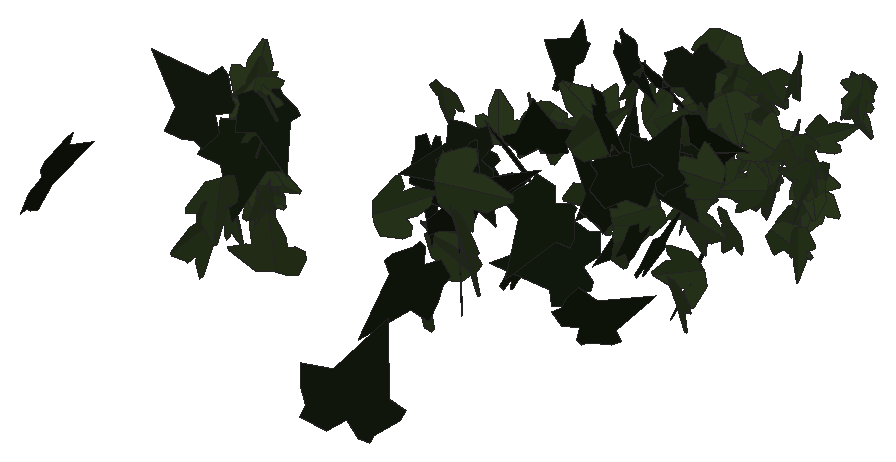
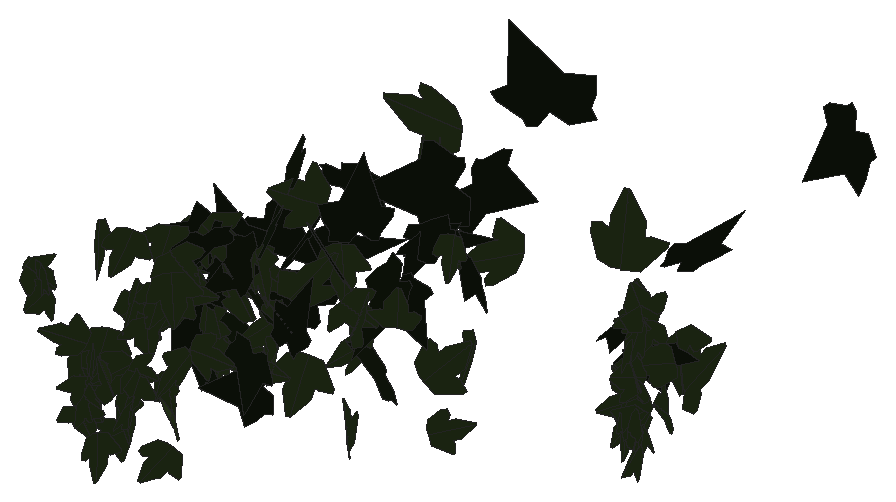
# SketchUp Ruby script. Lengths in inches.
U = 1.inch
M = Sketchup.active_model
def pt(a) = Geom::Point3d.new(a.map { |v| v * U })
def face(e, loops, mat)
  f = e.add_face(loops[0].map { |a| pt(a) })
  loops[1..].each { |l| e.add_face(l.map { |a| pt(a) }).erase! }
  f.material = f.back_material = mat if mat
  f
end
# faces: each face lists its corners as indices into pts; further lists are holes
def faces(e, pts, list, mat = nil) = list.each { |f| face(e, (f[0].is_a?(Array) ? f : [f]).map { |l| l.map { |i| pts[i] } }, mat) }
# xy, xz, yz: faces in a plane at the given z, y or x. An outline is a flat list of corners, or four numbers for a rectangle; further outlines are holes
def ring(l) = l.size == 4 ? [[l[0], l[1]], [l[2], l[1]], [l[2], l[3]], [l[0], l[3]]] : l.each_slice(2).to_a
def flat(e, list, mat, &to3) = list.each { |f| face(e, (f[0].is_a?(Array) ? f : [f]).map { |l| ring(l).map { |u, v| to3.(u, v) } }, mat) }
def xy(e, z, list, mat = nil) = flat(e, list, mat) { |x, y| [x, y, z] }
def xz(e, y, list, mat = nil) = flat(e, list, mat) { |x, z| [x, y, z] }
def yz(e, x, list, mat = nil) = flat(e, list, mat) { |y, z| [x, y, z] }
def lines(e, pts, list) = list.each { |a, b| e.add_line(pt(pts[a]), pt(pts[b])) }
# prism: a flat outline (further loops are holes) pulled along v
def prism(e, loops, v, mat = nil)
  f = face(e, loops, mat); d = Geom::Vector3d.new(v.map { |x| x * U })
  f.pushpull(f.normal.samedirection?(d) ? d.length : -d.length)
end
def box(e, o, s, mat = nil) = prism(e, [[o, [o[0] + s[0], o[1], o[2]], [o[0] + s[0], o[1] + s[1], o[2]], [o[0], o[1] + s[1], o[2]]]], [0, 0, s[2]], mat)
def at(x, y, z, deg = 0) = Geom::Transformation.translation(pt([x, y, z])) * Geom::Transformation.rotation(ORIGIN, Z_AXIS, deg.degrees)
def axes(o, x, y, z) = Geom::Transformation.new([*x, 0, *y, 0, *z, 0, *pt(o).to_a, 1])
def part(name) = M.definitions.add(name)
# library, detail: a bought-in or finely detailed component or shape, given as its bounding box
def library(name, o, s) = part(name).tap { |d| box(d.entities, o, s) }
def detail(e, o, s) = box(e.add_group.entities, o, s)
def put(e, d, t, mat = nil) = e.add_instance(d, t).tap { |i| i.material = mat if mat }
def group(e, t, mat = nil) = e.add_group.tap { |g| g.transformation = t; g.material = mat if mat }.entities
root = M.entities
M.materials.add("efeu1").color = [18, 25, 13]
M.materials.add("efeu2").color = [43, 57, 29]
c1 = part("ivyleaf_10")
p = [[0,0.5,-0.03],[-0.0625,2.02,-0.43],[-0.19,2.01,-0.46],[-0.54,1.05,-0.29],[-0.52,0.625,-0.18],[-0.83,0.76,-0.28],
  [-1.16,0.64,-0.33],[-1.15,0.33,-0.24],[-0.77,-0.39,0.02],[-0.3,-0.51,0.16],[0.04,-0.48,0.23],[-0.02,2.01,-0.4375],
  [-0.06,2.01,-0.43],[0.04,-0.49,0.23],[0.67,-0.49,0.14],[1.38,0.36,-0.2],[1.375,0.51,-0.24],[0.81,0.65,-0.19],
  [0.62,0.59,-0.15],[0.6,1.09,-0.28],[0.5,1.23,-0.31]]
faces(c1.entities,p,[[0,1,2,3,4,5,6,7,8,9,10],[11,12,0,13,14,15,16,17,18,19,20]],"efeu2")
c2 = part("ivyleaf_9")
p = [[1.54,2.16,1.25],[1.36,2.04,1.19],[-0.21,0.99,0.68],[-0.71,1.11,0.82],[-0.85,0.86,0.67],[-0.8,0.17,0.21],
  [-0.9,-0.01,0.1],[-0.67,-0.16,-0.02],[-0.08,-0.08,-0.05],[-0.03,-0.6,-0.4],[0.65,-0.88,-0.66],[0.83,-0.6,-0.49],
  [1.29,-0.42,-0.43],[1.8125,-0.07,-0.26],[1.21,0.44,0.15]]
faces(c2.entities,p,[[0,1,2,3,4,5,6,7,8,9,10,11,12,13,14]],"efeu1")
put(root,c1,axes([585.76,128.17,162.25],[-0.17005,-0.68524,-0.06078],[0.01227,-0.06562,0.70548],[-0.68782,0.16825,0.02761]))
put(root,c1,axes([585.82,127.98,162.4],[0.37144,0.64539,-0.33053],[0.14686,0.29672,0.7444],[0.71007,-0.39897,0.01894]))
put(root,c2,axes([586.1,116.46,164.15],[-0.29886,0.48619,-0.98361],[-0.5513,0.81487,0.57029],[0.94865,0.62673,0.02154]))
put(root,c1,axes([586.01,128.02,157.12],[0.06596,-0.11263,-0.71846],[-0.05388,0.71867,-0.11761],[0.72524,0.06363,0.05661]))
put(root,c1,axes([585.97,128.1875,160],[0.0874,-0.33565,0.67412],[-0.16899,0.65259,0.34684],[-0.73385,-0.19025,0.00041]))
put(root,c2,axes([586.45,125.03,162.97],[-0.48659,-0.88874,-0.04131],[-0.00959,-0.04184,1.01316],[-0.88965,0.48655,0.01168]))
put(root,c1,axes([585.93,128.22,161.91],[-0.67581,0.38769,-0.11767],[0.09092,-0.07788,-0.7788],[-0.39482,-0.68154,0.02206]))
put(root,c1,axes([585.39,127.52,160.49],[0.15739,0.12437,0.84893],[0.67828,0.51053,-0.20054],[-0.52544,0.69629,-0.00459]))
put(root,c1,axes([585.76,128,161.98],[0.63059,0.32559,0.23143],[0.20628,0.10493,-0.70968],[-0.34207,0.66347,-0.00134]))
put(root,c1,axes([585.85,128.32,158.59],[0.22534,0.43352,0.43267],[0.15933,0.40366,-0.48744],[-0.59141,0.27393,0.03354]))
put(root,c1,axes([586.08,128.1875,161.01],[-0.02766,-0.67059,0.01012],[0.11743,-0.01481,-0.66072],[0.66031,-0.02546,0.11793]))
put(root,c2,axes([586.01,127.55,160.63],[-0.54627,-0.74339,-0.23752],[0.15721,0.17916,-0.9223],[0.76441,-0.56809,0.01994]))
put(root,c1,axes([586.04,128.19,160.33],[0.36188,-0.4919,0.18543],[0.10622,-0.15206,-0.61065],[0.51484,0.37712,-0.00436]))
put(root,c1,axes([585.68,128.68,158.08],[-0.19949,0.03059,0.62859],[0.62716,-0.04513,0.20123],[0.05229,0.65794,-0.01542]))
put(root,c1,axes([585.99,127.93,158.08],[0.57753,-0.32477,0.3316],[0.29454,-0.15268,-0.6625],[0.35872,0.64822,0.0101]))
put(root,c1,axes([585.74,126.84,158.2],[0.19568,-0.09663,0.72486],[0.6784,-0.25615,-0.21728],[0.27301,0.70576,0.02038]))
put(root,c1,axes([586.19,125.04,158.41],[0.02125,-0.04855,-1.12887],[-0.07201,-1.12683,0.0471],[-1.12761,0.07105,-0.02428]))
put(root,c1,axes([586.32,128.14,158.55],[0.08546,-0.76323,-0.25848],[0.08378,0.26694,-0.7605],[0.80144,0.05347,0.10706]))
put(root,c1,axes([585.96,128.17,159.27],[0.47558,-0.01667,-0.43561],[0.43518,-0.01957,0.47587],[-0.02551,-0.64463,-0.00318]))
put(root,c1,axes([585.99,128.17,159.18],[-0.34314,-0.0798,-0.64142],[0.62697,0.1355,-0.35227],[0.15718,-0.71471,0.00483]))
put(root,c1,axes([586.42,125.37,159.8125],[-0.12869,-0.94375,0.15344],[0.22453,-0.18032,-0.92078],[0.9294,-0.08711,0.24369]))
put(root,c2,axes([586.36,127.99,161.99],[0.09162,-0.82395,-0.25375],[0.09024,0.26294,-0.82121],[0.8574,0.06038,0.11354]))
put(root,c1,axes([591.375,122.16,160.26],[-1.00306,-0.38729,-0.06213],[-0.05798,-0.02233,1.07523],[-0.38793,1.00473,-0.00005]))
put(root,c1,axes([591.79,131.49,157.33],[-0.16698,-0.03358,-0.619],[-0.59143,-0.18344,0.16949],[-0.18574,0.61432,0.01678]))
put(root,c1,axes([592.43,130.02,163.62],[-0.62546,0.09653,0.09939],[-0.09815,0.01567,-0.63286],[-0.0978,-0.63311,-0.00051]))
put(root,c1,axes([593.05,132.11,161.41],[0.63703,0.33089,0.02154],[-0.01915,-0.00988,0.71784],[0.33103,-0.63732,0.00006]))
put(root,c1,axes([593.84,129.17,157.85],[-0.5698,-0.12119,-0.60933],[-0.58442,-0.17597,0.5815],[-0.21079,0.81547,0.03493]))
put(root,c2,axes([593.03,128.44,162.24],[-0.5686,-0.00907,-0.92129],[0.92126,0.00792,-0.56866],[0.0115,-1.08259,0.00356]))
put(root,c1,axes([593.25,125.9,161.16],[-0.01945,-0.10977,0.97653],[0.15156,0.96469,0.11146],[-0.97092,0.15279,-0.00217]))
put(root,c1,axes([594.14,126.85,157.52],[-0.09548,0.17171,0.87506],[-0.55339,0.67869,-0.19356],[-0.69926,-0.56056,0.0337]))
put(root,c1,axes([594.06,133.03,161.12],[-0.48533,0.59394,-0.20512],[-0.14599,0.14551,0.76675],[0.61117,0.5064,0.02027]))
put(root,c2,axes([594.72,128.85,162.4],[-0.53318,-0.26031,0.69488],[-0.62759,-0.29836,-0.59331],[0.39592,-0.82348,-0.00469]))
put(root,c1,axes([594.33,133.15,162.02],[0.35419,0.50006,-0.52363],[-0.30425,-0.42617,-0.61279],[-0.65702,0.46692,0.00148]))
put(root,c2,axes([594,130.97,161.95],[0.95256,-0.13069,-0.37223],[-0.36291,0.0912,-0.96072],[0.15471,1.01863,0.03826]))
put(root,c2,axes([594.65,130.04,161.18],[0.24765,0.36355,-0.63218],[-0.35693,-0.52178,-0.43988],[-0.63594,0.43443,0.0007]))
put(root,c2,axes([595.06,133.55,164.09],[-0.3395,0.47589,0.60779],[-0.36012,0.48966,-0.58455],[-0.68279,-0.49488,0.00609]))
put(root,c1,axes([594.28,133.09,156.81],[-0.35362,0.21173,0.70281],[0.61625,-0.33818,0.41194],[0.39877,0.71037,-0.01336]))
put(root,c2,axes([594.52,128.42,162.52],[0.10169,-0.67946,-0.53104],[-0.05019,0.52915,-0.68665],[0.8609,0.11111,0.02269]))
put(root,c2,axes([595.32,130.03,157.63],[-0.42986,0.75206,0.02487],[-0.00351,-0.03065,0.86605],[0.75246,0.42949,0.01825]))
put(root,c1,axes([595.82,131.68,162.71],[-0.73307,-0.23476,0.16603],[-0.15728,-0.05326,-0.76974],[0.24071,-0.74975,0.00269]))
put(root,c2,axes([595.81,134.46,160.8],[0.50022,-0.44274,0.48734],[-0.29427,0.39717,0.66287],[-0.589,-0.57443,0.0827]))
put(root,c1,axes([595.9375,133.6875,162.22],[0.36772,0.64982,0.52167],[-0.26433,-0.4498,0.74662],[0.79028,-0.45281,0.00699]))
put(root,c1,axes([595.77,133.71,159.37],[-0.82903,-0.26842,-0.15135],[0.14547,0.04205,-0.87139],[0.27166,-0.84168,0.00473]))
put(root,c1,axes([596.06,130.25,158.64],[-0.01568,0.00241,0.85392],[-0.14335,0.84193,-0.00501],[-0.8418,-0.14342,-0.01505]))
put(root,c1,axes([596.625,138.13,161.61],[0.02824,0.03695,-0.70207],[-0.67647,0.19278,-0.01706],[0.19146,0.67567,0.04326]))
put(root,c2,axes([596.65,135.32,160.22],[-0.01499,0.73208,0.27968],[-0.00057,0.27972,-0.73221],[-0.78368,-0.01421,-0.00481]))
put(root,c2,axes([596.32,130.07,162.95],[0.6793,0.26432,0.44165],[-0.43261,-0.10302,0.72705],[0.27887,-0.80367,0.05206]))
put(root,c2,axes([596.11,125.47,162.57],[0.08963,0.84283,-0.82162],[-0.00034,0.82402,0.84525],[1.17704,-0.06394,0.06281]))
put(root,c2,axes([596.35,135.3125,159.11],[0.00938,0.60199,-0.51412],[-0.01729,0.51419,0.60175],[0.79146,0.0041,0.01924]))
put(root,c1,axes([596.6875,134.92,163.59],[0.19718,-0.7557,0.00758],[0.00996,-0.00523,-0.78095],[0.75567,0.19726,0.00832]))
put(root,c2,axes([596.44,134.51,164.77],[0.58554,-0.44412,-0.42017],[-0.32892,0.26158,-0.73487],[0.51536,0.67155,0.00837]))
put(root,c2,axes([596.8,123.27,161.42],[-0.03527,-0.00885,-1.11829],[0.41072,-1.04076,-0.00472],[-1.04018,-0.41066,0.03605]))
put(root,c1,axes([597.3125,134.75,159.25],[-0.06897,-0.06168,0.68232],[-0.51498,-0.44761,-0.09252],[0.45184,-0.51957,-0.0013]))
put(root,c2,axes([597.21,133.59,161.13],[-0.64791,0.38477,-0.14043],[-0.13274,0.05138,0.75319],[0.38749,0.66096,0.0232]))
put(root,c1,axes([596.9,133.97,159.58],[-0.37143,0.46703,-0.38856],[0.23089,-0.31274,-0.59661],[-0.56195,-0.43719,0.01169]))
put(root,c1,axes([596.91,135.45,161.93],[0.64924,-0.28052,-0.4279],[0.39089,-0.17413,0.70723],[-0.33014,-0.75782,-0.00412]))
put(root,c2,axes([596.93,135.23,163.6875],[0.78065,-0.20446,0.08123],[0.07855,-0.02069,-0.80698],[0.2055,0.78459,-0.00011]))
put(root,c1,axes([597.57,136.58,161.9],[0.10655,-0.55823,-0.51413],[-0.08967,0.50628,-0.56828],[0.7536,0.13917,0.00507]))
put(root,c1,axes([597.32,139.15,157.91],[-0.5087,-0.17584,-0.37285],[0.35164,0.12397,-0.53823],[0.21513,-0.61841,-0.00188]))
put(root,c1,axes([597.97,138.08,158.68],[0.44654,-0.018,0.5821],[-0.47995,0.40411,0.38067],[-0.32987,-0.61232,0.23412]))
put(root,c1,axes([597.8125,137.62,160.57],[-0.03237,0.42903,0.62238],[-0.09536,0.61565,-0.42935],[-0.74988,-0.09681,0.02773]))
put(root,c2,axes([597.26,124.625,162.97],[-0.16332,0.06873,-1.20253],[1.1576,-0.32635,-0.17587],[-0.33281,-1.16887,-0.02161]))
put(root,c1,axes([598.16,137.79,163.5],[-0.58024,-0.4564,0.07783],[-0.06659,-0.04122,-0.73818],[0.45818,-0.58398,-0.00872]))
put(root,c1,axes([597.09,124.5625,164.2],[0.06794,-0.03429,-1.21752],[1.19708,-0.22315,0.07308],[-0.22477,-1.19882,0.02122]))
put(root,c1,axes([598.26,137.43,164.35],[0.44897,0.50651,-0.3677],[-0.27339,-0.24837,-0.67594],[-0.56304,0.52449,0.035]))
put(root,c1,axes([597.99,130.45,163.48],[-0.01164,-0.515,0.77856],[0.12607,0.77062,0.51164],[-0.92493,0.11152,0.05994]))
put(root,c1,axes([598.5,137.09,162.6875],[-0.2274,-0.03849,0.70203],[-0.2665,-0.67806,-0.1235],[0.65062,-0.29119,0.19478]))
put(root,c1,axes([598.17,123.57,163.4],[-0.83234,0.7442,-0.39698],[0.28754,-0.27396,-1.11646],[-0.79294,-0.88053,0.01185]))
put(root,c2,axes([598.67,130.81,161.18],[-0.06434,-0.83718,0.30362],[0.02164,0.30285,0.83965],[-0.89028,0.06786,-0.00153]))
put(root,c1,axes([598.46,131.88,159.36],[-0.02442,-0.07854,-0.94323],[0.26238,0.906,-0.08224],[0.9094,-0.26351,-0.0016]))
put(root,c2,axes([598.3,135.88,164.44],[-0.05154,-0.68036,-0.38634],[0.07391,0.38122,-0.68119],[0.7789,-0.08119,0.03908]))
put(root,c1,axes([598.6,137.875,163.08],[-0.51475,-0.34601,-0.14546],[0.1217,0.0797,-0.62023],[0.35507,-0.52893,0.0017]))
put(root,c1,axes([598.48,137.3,162.66],[-0.43045,-0.48124,-0.35068],[0.32947,0.16796,-0.6349],[0.49601,-0.5292,0.1174]))
put(root,c2,axes([598.56,130.48,164.99],[0.67111,-0.30019,-0.61332],[-0.54798,0.27635,-0.73486],[0.40743,0.86613,0.02189]))
put(root,c2,axes([599.18,132.04,160.2],[-0.84412,0.47718,-0.05622],[0.04814,-0.02908,-0.96966],[-0.47806,-0.84549,0.00162]))
put(root,c2,axes([599.32,128.54,160.08],[-0.43789,-0.1826,0.92619],[-0.859,-0.34637,-0.47441],[0.39152,-0.96416,-0.00498]))
put(root,c2,axes([599.25,135.08,161.8],[-0.698,-0.01688,0.31629],[-0.31621,-0.00719,-0.6982],[0.01834,-0.76628,-0.00042]))
put(root,c2,axes([599.16,127.3,162.84],[-0.90542,-0.38283,-0.11285],[0.10356,0.04485,-0.98303],[0.38544,-0.91133,-0.00097]))
put(root,c1,axes([598.97,136.0625,162.59],[-0.2696,-0.6822,-0.18443],[0.12193,0.14953,-0.73134],[0.69609,-0.29041,0.05668]))
put(root,c1,axes([598.91,138.14,161.89],[0.37797,0.62121,-0.07646],[-0.06493,-0.04992,-0.72657],[-0.62252,0.38238,0.02936]))
put(root,c1,axes([598.84,137.32,162.99],[0.04211,-0.21788,-0.6056],[0.08872,-0.59914,0.22172],[-0.63746,-0.09778,-0.00915]))
put(root,c1,axes([599.05,138.6875,160.3],[0.19223,0.36446,-0.49963],[-0.21327,-0.45204,-0.41181],[-0.58049,0.28677,-0.01415]))
put(root,c2,axes([599.37,131.19,162.61],[0.05985,0.23906,-0.85319],[-0.14741,-0.84053,-0.24586],[-0.8737,0.15819,-0.01696]))
put(root,c1,axes([599.72,131.73,161.04],[-0.34902,-0.10855,0.79418],[-0.65593,-0.45919,-0.35103],[0.46072,-0.73599,0.10187]))
put(root,c1,axes([599.11,138.75,159.76],[-0.50773,-0.42061,-0.14316],[0.21742,-0.04563,-0.63706],[0.38748,-0.52555,0.16988]))
put(root,c1,axes([599.13,138.8125,158.91],[-0.08675,0.61072,-0.17549],[0.02758,-0.17333,-0.61684],[-0.63483,-0.09098,-0.00282]))
put(root,c2,axes([599.2,132.35,158.47],[-0.38495,0.87411,-0.002],[-0.02444,-0.00858,0.95477],[0.87377,0.38486,0.02582]))
put(root,c2,axes([599.36,134.97,161.01],[0.2706,0.7053,0.15299],[0.04742,0.14566,-0.75539],[-0.72014,0.27461,0.00775]))
put(root,c1,axes([599.57,133.89,163.24],[-0.14524,-0.64406,0.54774],[-0.11227,-0.53615,-0.6602],[0.83799,-0.18346,0.00649]))
put(root,c1,axes([599.7,134.39,159.98],[-0.48082,-0.3359,-0.51431],[-0.36437,-0.36987,0.58221],[-0.49455,0.59908,0.07108]))
put(root,c1,axes([599.77,136.05,158.41],[-0.56897,0.22339,0.37456],[-0.38275,0.03937,-0.60488],[-0.20906,-0.68005,0.08802]))
put(root,c1,axes([599.5625,138.49,158.75],[0.06911,-0.65577,-0.06218],[-0.00554,0.06194,-0.6594],[0.65869,0.06933,0.00098]))
put(root,c2,axes([599.29,132.9,161.97],[0.11258,-0.5372,-0.63452],[-0.04902,0.63491,-0.54623],[0.82994,0.11038,0.05381]))
put(root,c1,axes([599.54,134.88,162.97],[-0.4859,0.67819,-0.15707],[0.08208,-0.1344,-0.83421],[-0.69129,-0.49265,0.01136]))
put(root,c1,axes([599.33,138.8125,160.37],[-0.44365,-0.03239,-0.53298],[0.53239,0.02646,-0.44476],[0.04107,-0.69296,0.00793]))
put(root,c1,axes([599.62,139.3,159.65],[0.23611,-0.6075,0.09977],[-0.03246,0.09443,0.65175],[-0.61478,-0.2383,0.0039]))
put(root,c1,axes([599.81,139.64,157.65],[-0.18805,-0.59673,-0.12491],[0.01472,0.12623,-0.62522],[0.60948,-0.18716,-0.02343]))
put(root,c1,axes([599.8,137.54,162.51],[0.11529,-0.50236,-0.55334],[0.00749,0.56063,-0.50742],[0.74732,0.07188,0.09045]))
put(root,c1,axes([599.54,134.38,160.4],[0.19748,-0.34368,0.67317],[0.36934,-0.56316,-0.39587],[0.65944,0.41834,0.02012]))
put(root,c2,axes([599.56,132.1875,162.04],[-0.5493,0.21702,0.62365],[0.53355,-0.33209,0.5855],[0.38905,0.76183,0.07757]))
put(root,c2,axes([599.63,115.79,160.07],[-0.86198,-0.07692,0.96033],[0.95858,-0.19731,0.8446],[0.09632,1.27527,0.18861]))
put(root,c1,axes([600.65,132.85,158.45],[0.37804,-0.0153,-0.80151],[-0.77702,0.21099,-0.37051],[0.1972,0.8607,0.07658]))
put(root,c1,axes([600.41,137.07,161.39],[0.17615,0.46603,0.56658],[-0.26195,-0.50431,0.49626],[0.68526,-0.31258,0.04406]))
put(root,c2,axes([600.33,133.7,158.35],[-0.50735,0.32333,-0.48682],[0.38976,-0.29315,-0.6009],[-0.43545,-0.6391,0.02935]))
put(root,c1,axes([600.29,132.375,157.9],[-0.69547,0.46011,-0.04222],[0.03263,-0.0272,-0.83389],[-0.46089,-0.69622,0.00467]))
put(root,c2,axes([599.67,128.25,158.04],[0.12904,-0.08419,0.94172],[0.94015,0.11211,-0.1188],[-0.10016,0.94388,0.0981]))
put(root,c1,axes([599.6875,134.26,159.53],[0.00552,-0.02259,-0.88683],[0.76033,-0.45677,0.01637],[-0.45703,-0.76017,0.01652]))
put(root,c2,axes([599.7,134.05,162.86],[0.43893,-0.14346,0.62728],[0.59279,-0.20524,-0.46173],[0.25033,0.73757,-0.00648]))
put(root,c1,axes([600.11,138.25,157.3],[-0.37729,-0.06423,-0.52016],[0.51952,0.03877,-0.38162],[0.06918,-0.64141,0.02902]))
put(root,c1,axes([600.27,135.25,163.62],[0.43588,0.56842,0.17247],[0.10413,0.13749,-0.71631],[-0.58481,0.44815,0.001]))
put(root,c1,axes([601.1,133.24,161.98],[0.15101,0.12074,0.8499],[-0.69327,-0.49174,0.19304],[0.50624,-0.70945,0.01084]))
put(root,c1,axes([600.62,139.24,158.84],[-0.06252,0.54809,-0.35241],[-0.18215,-0.35461,-0.51921],[-0.62564,0.04847,0.18638]))
put(root,c1,axes([600.5625,138.33,160.8125],[-0.49451,-0.47064,-0.21459],[0.18201,0.11957,-0.68166],[0.48417,-0.52563,0.03708]))
put(root,c1,axes([600.83,136.06,160.2],[0.03665,0.20392,0.67379],[-0.10685,-0.66527,0.20716],[0.69581,-0.1129,-0.00368]))
put(root,c1,axes([600.66,136.95,163.96],[-0.48658,-0.39577,-0.2622],[0.20845,0.15923,-0.62717],[0.42653,-0.5293,0.00739]))
put(root,c1,axes([601.25,138.68,159.68],[0.03986,0.04852,-0.64974],[-0.6513,0.02068,-0.03841],[0.01773,0.65063,0.04968]))
put(root,c1,axes([600.83,139.35,158.4],[0.54009,0.29952,-0.17926],[-0.14542,-0.10715,-0.61718],[-0.31733,0.55888,-0.02226]))
put(root,c1,axes([600.85,138.99,159.3],[0.47324,0.47123,0.07495],[0.05422,0.05178,-0.66784],[-0.47406,0.47633,-0.00156]))
put(root,c1,axes([601.24,138.61,160.01],[-0.24237,-0.60548,0.22694],[-0.07948,-0.21263,-0.65217],[0.64171,-0.25502,0.00495]))
put(root,c1,axes([600.97,138.68,160.44],[-0.48307,0.34353,-0.33091],[0.19792,-0.28416,-0.58391],[-0.43398,-0.51197,0.10205]))
put(root,c1,axes([601.35,137.58,164.29],[0.23278,-0.67396,-0.27143],[0.0244,0.29211,-0.70439],[0.72615,0.20623,0.11068]))
put(root,c1,axes([601.07,139.1875,160.95],[-0.14902,-0.1891,0.59768],[0.38071,0.46077,0.2407],[-0.49804,0.4088,0.00516]))
put(root,c1,axes([601.64,137.35,158.06],[-0.08597,0.66245,-0.25128],[0.01613,-0.25123,-0.66783],[-0.70832,-0.08612,0.01529]))
put(root,c1,axes([602.45,139.55,163.3],[-0.58481,0.21974,-0.13617],[0.04764,-0.23945,-0.59095],[-0.25408,-0.55065,0.20263]))
put(root,c1,axes([602.22,139.53,162.49],[-0.50192,0.06422,-0.3958],[0.37035,-0.16882,-0.49704],[-0.15369,-0.61651,0.09488]))
put(root,c1,axes([602.62,139.6,163.24],[-0.1473,-0.41469,0.46308],[-0.00049,-0.47582,-0.42626],[0.62162,-0.09864,0.10939]))
